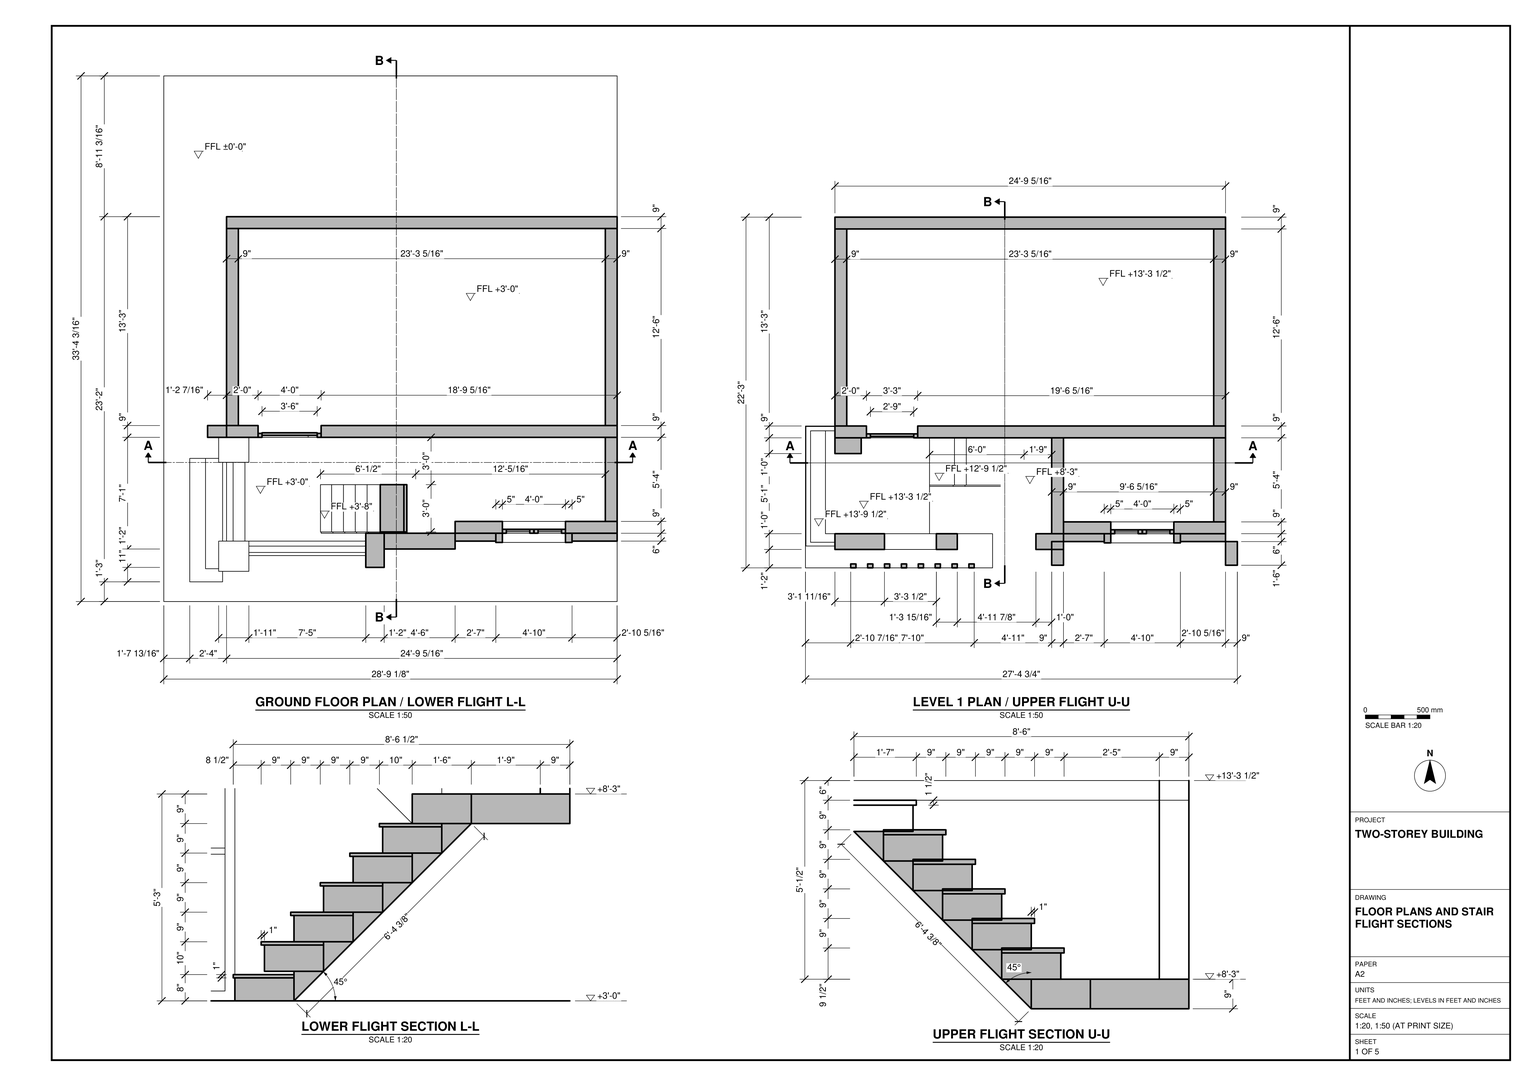
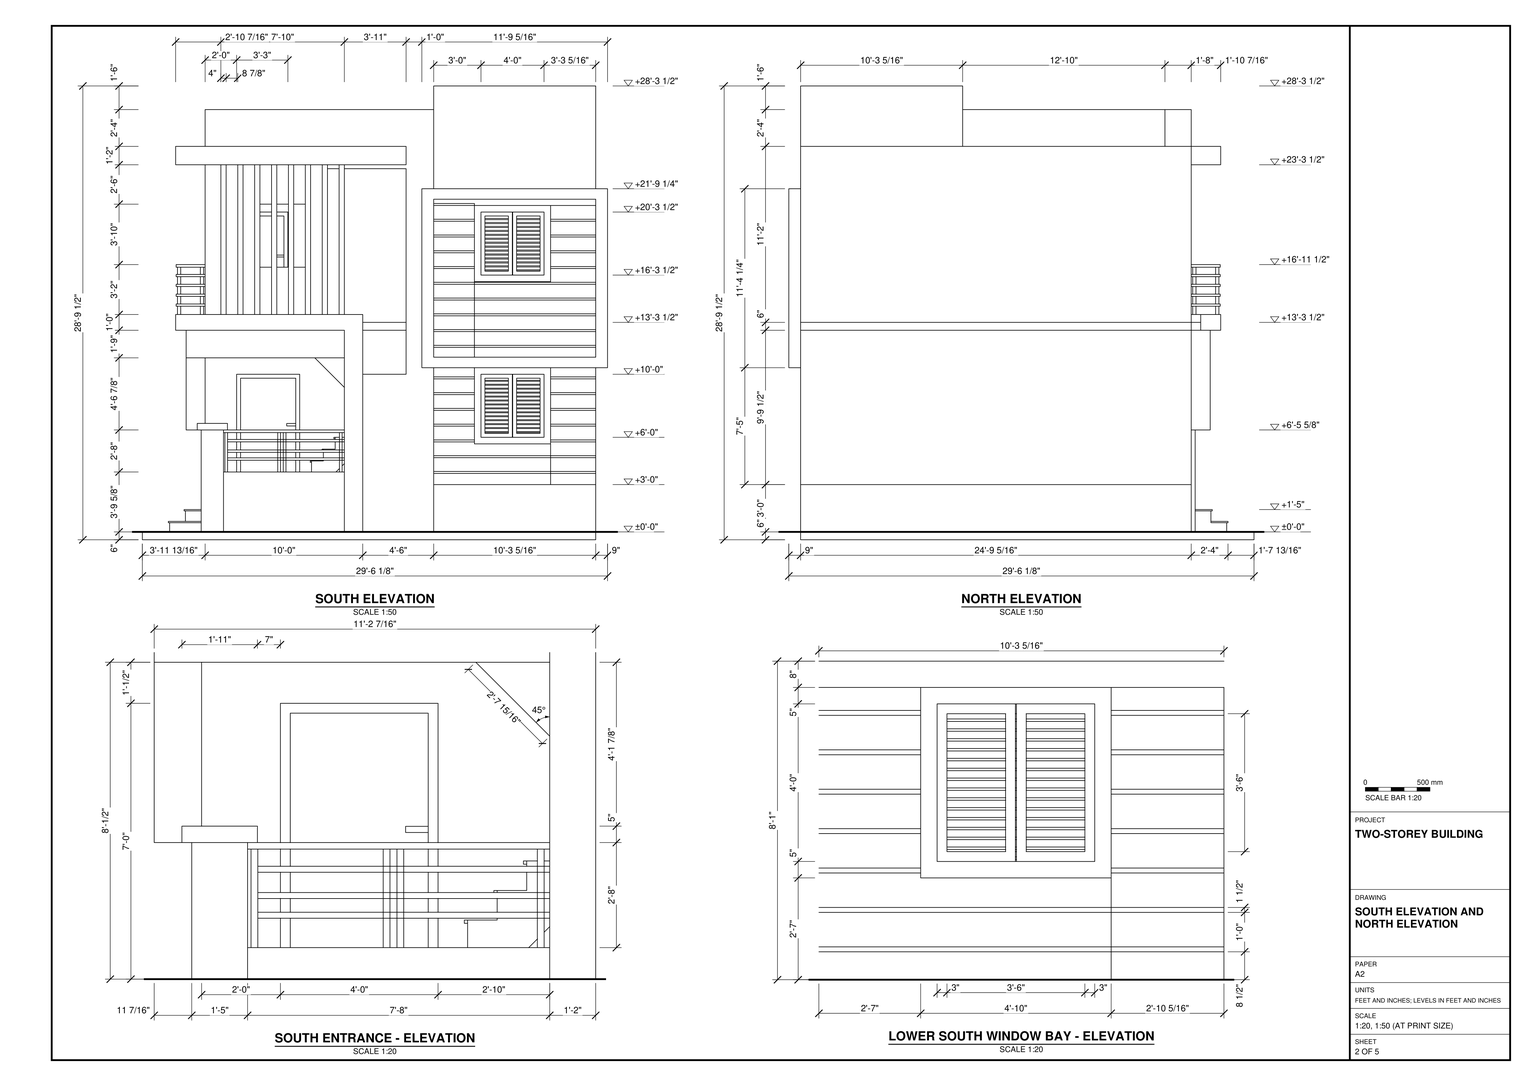
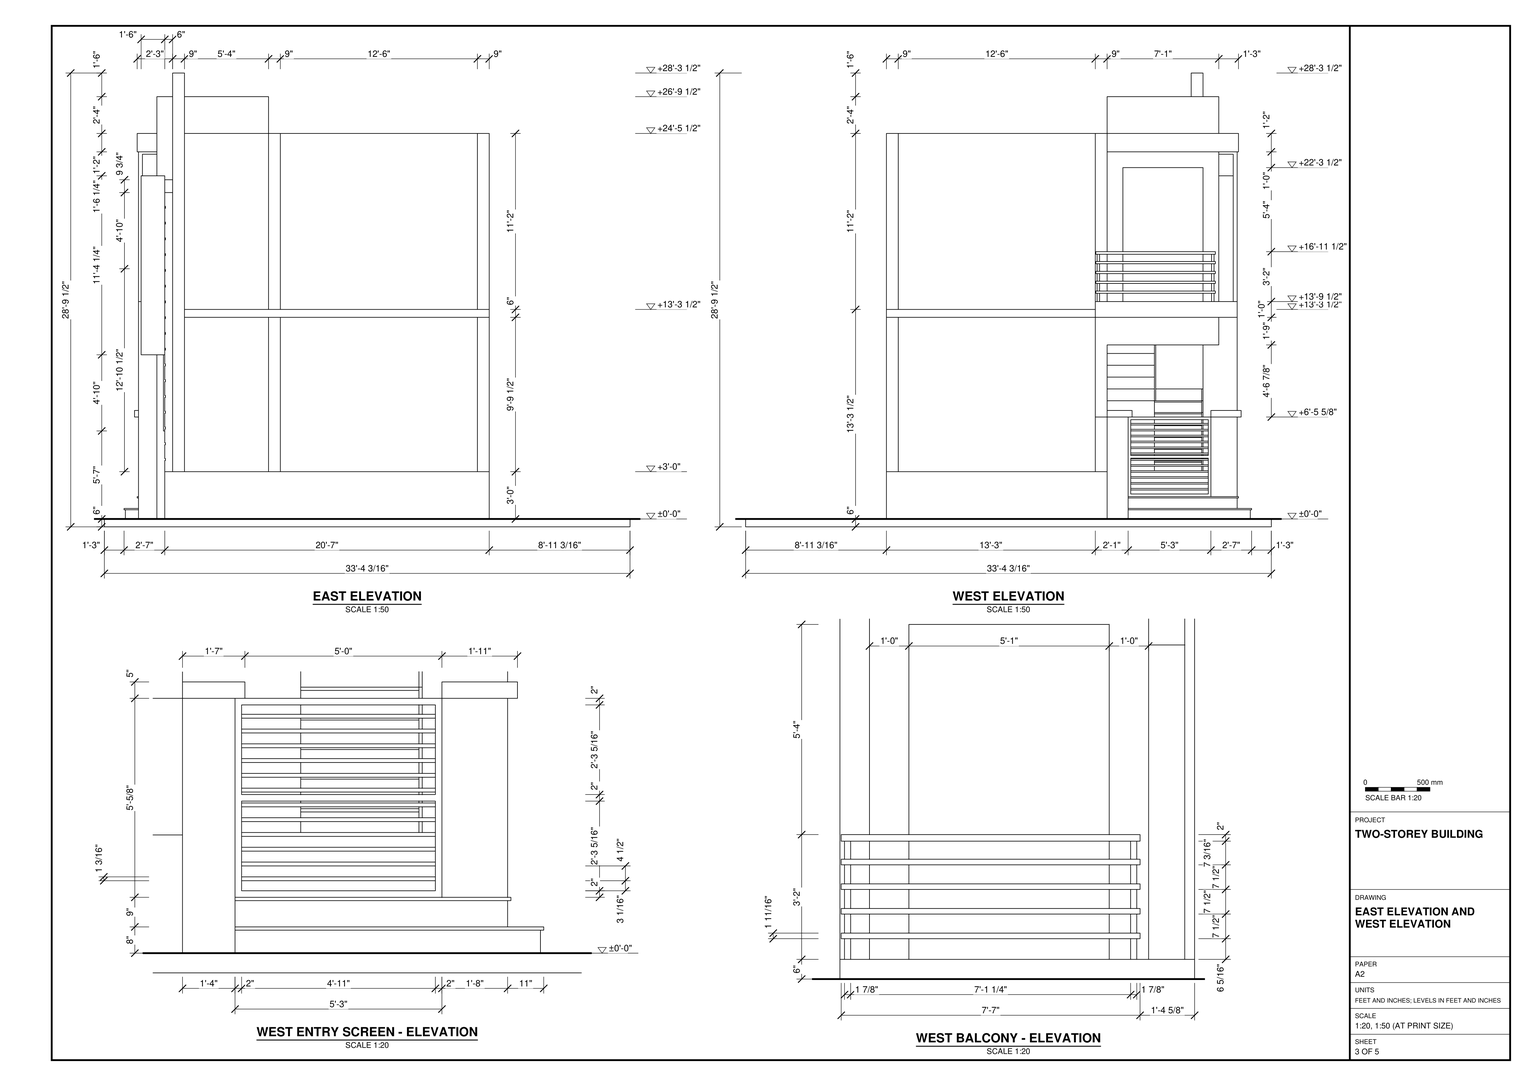
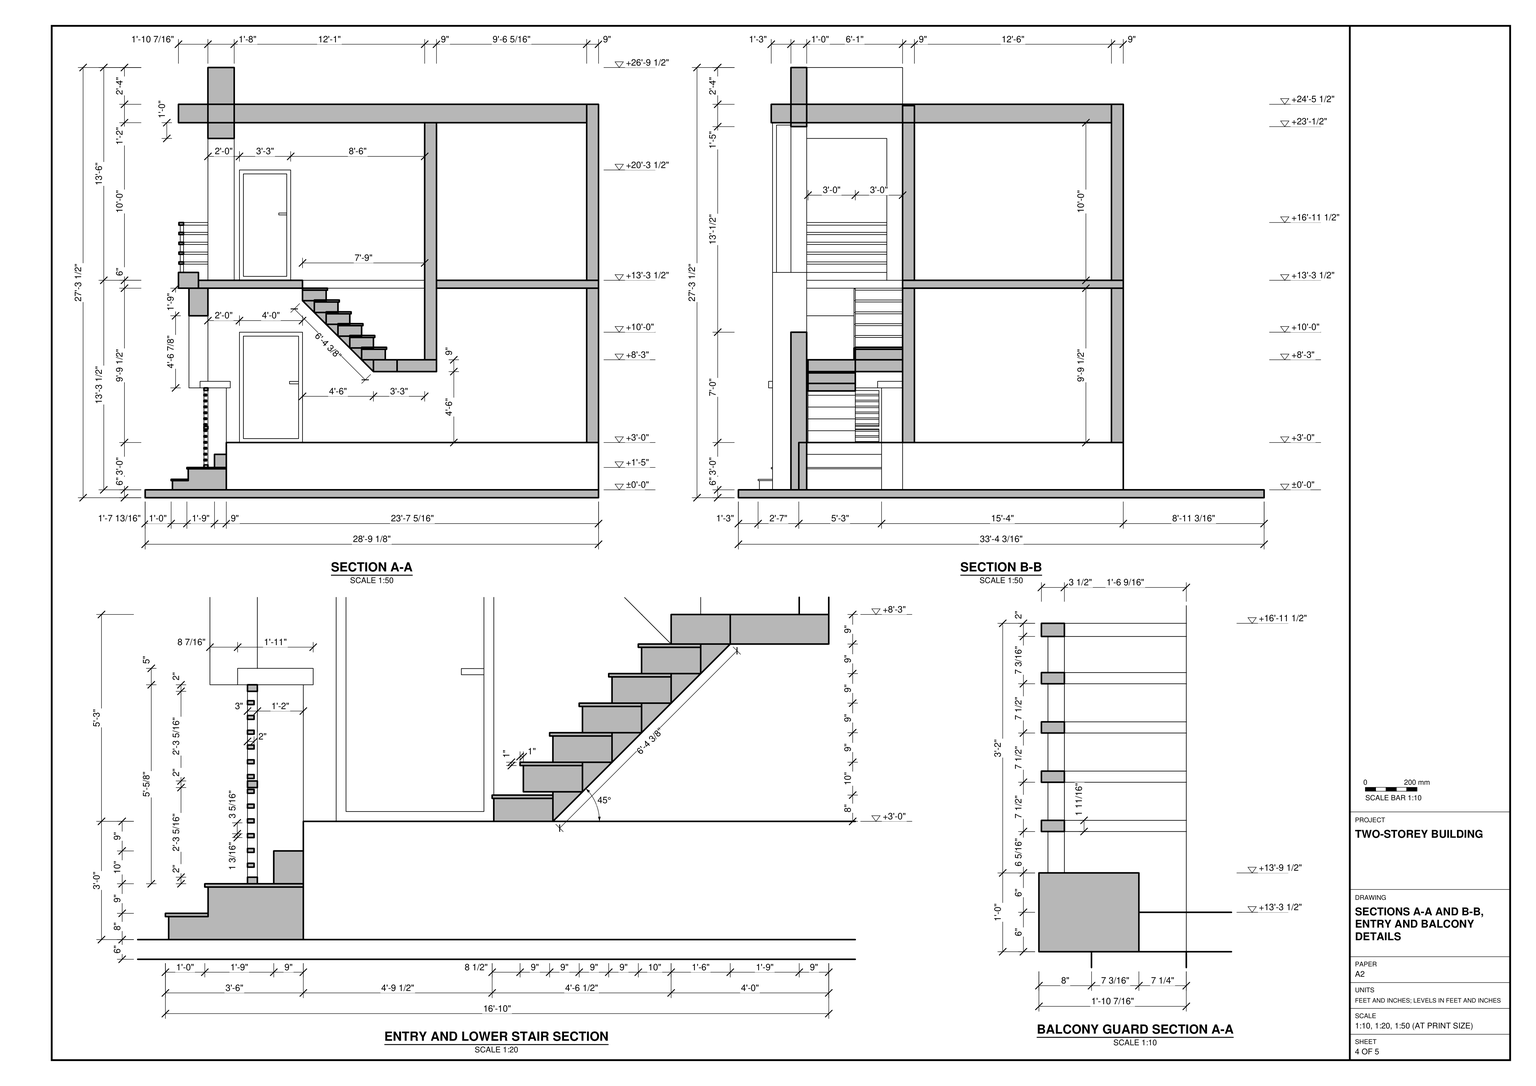
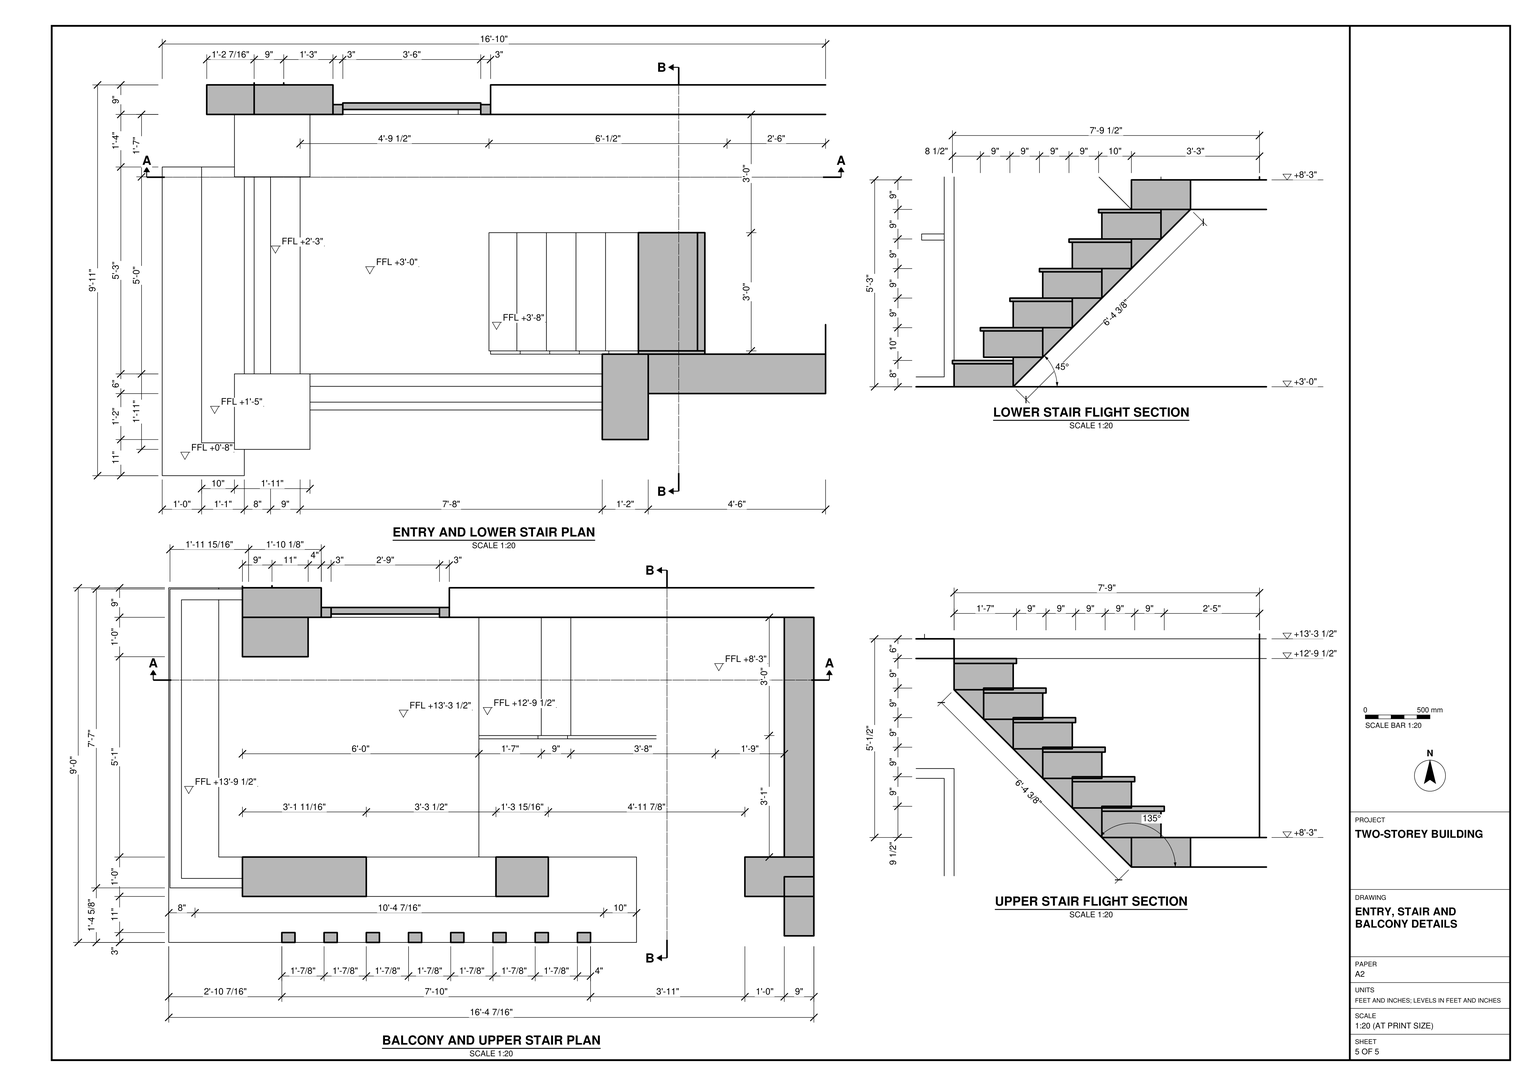
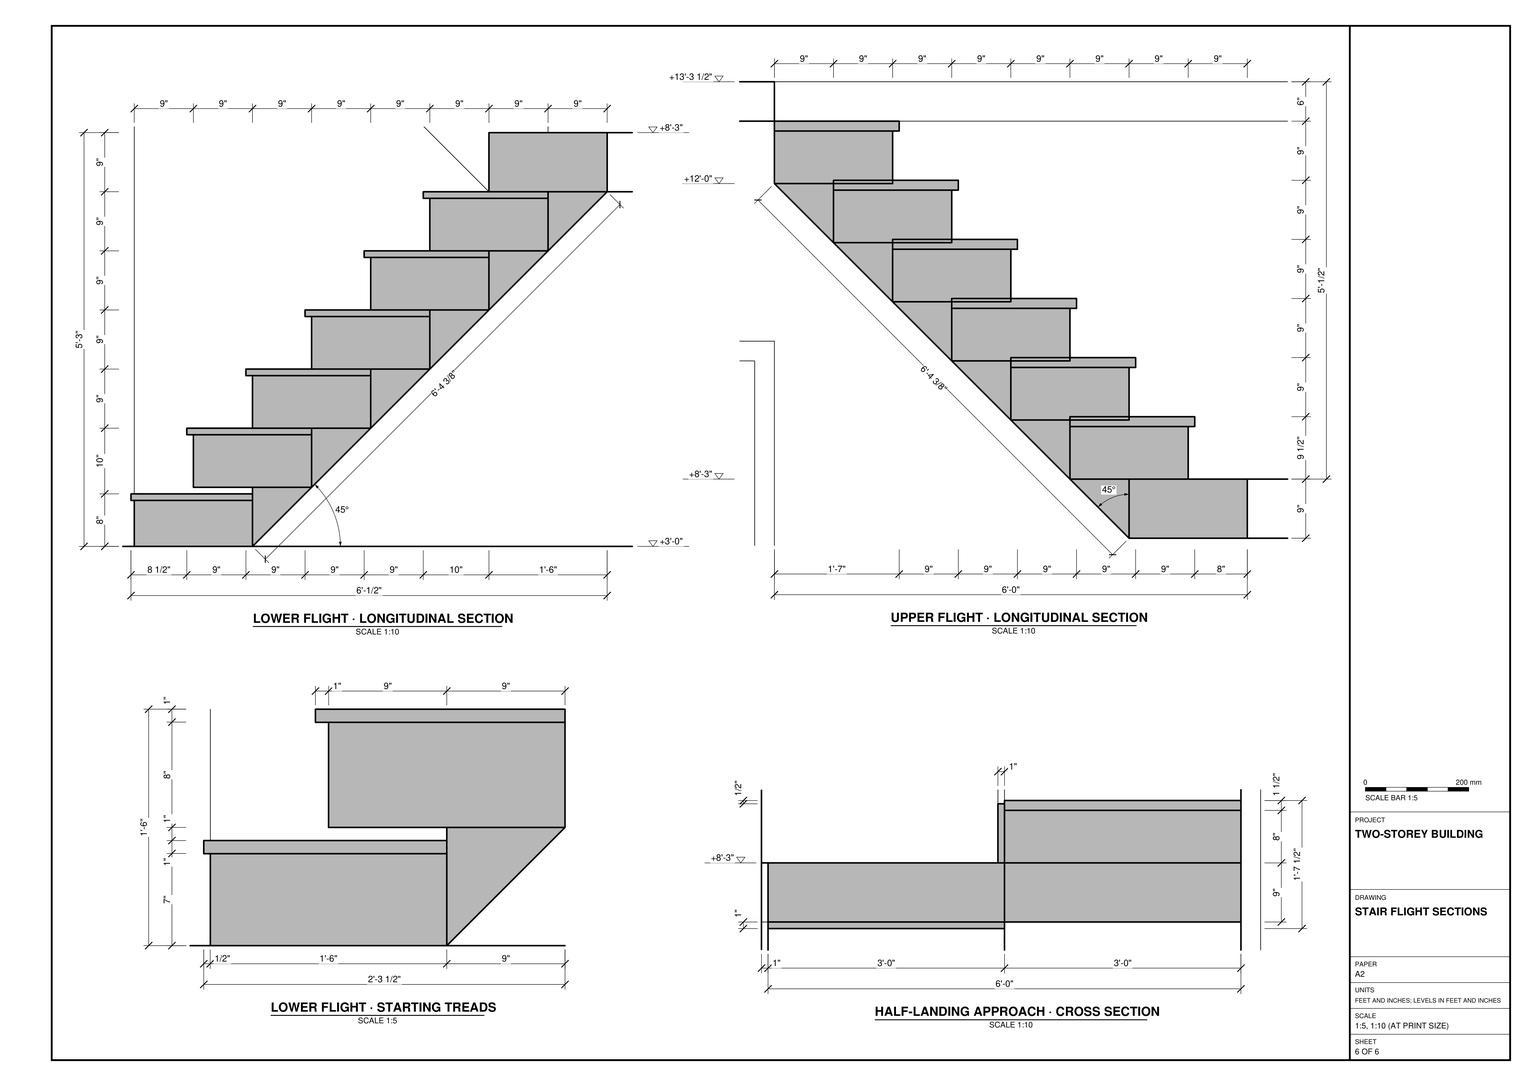
Build the two-storey building in SketchUp from task_files/diagram_01.pdf. Work in feet and inches. Set the overall width to 29'-6 1/8", depth to 33'-4 3/16" and height to 28'-9 1/2", including the base slab and projecting facade elements. Use ±0'-0" as the ground datum and +13'-3 1/2" as the upper storey level. Distinguish the ground datum from the raised lower floor at +3'-0".

Lay out the rectangular rear enclosure and the entrance, stair and window bay along its south side. Follow the wall thicknesses in plan, including the 9" walls around the rear enclosure. Model the base, raised floor, upper slab, balcony supports and flat roof profile with its changes in height. Use the flight sections to build the stair treads and risers, with the lower flight rising to the landing at +8'-3" and the upper flight returning to the upper floor.

Use the entrance and balcony details to position the steps, posts, horizontal rails and screens around the door openings. On the south window bay, model the stacked window units, horizontal bands and projecting upper surround. Keep the north elevation plain as drawn. Decor and loose items, if included, may be any suitable library components.

Keep shell elements such as walls, slabs and roof, and each furniture or joinery piece, in separate groups or components. Use components for repeated parts. Save one SketchUp model as output_files/two_storey_building_with_a_return_stair_and_balcony.skp.

# SketchUp Ruby script. Lengths in inches.
U = 1.inch
M = Sketchup.active_model
def pt(a) = Geom::Point3d.new(a.map { |v| v * U })
def face(e, loops, mat)
  f = e.add_face(loops[0].map { |a| pt(a) })
  loops[1..].each { |l| e.add_face(l.map { |a| pt(a) }).erase! }
  f.material = f.back_material = mat if mat
  f
end
# faces: each face lists its corners as indices into pts; further lists are holes
def faces(e, pts, list, mat = nil) = list.each { |f| face(e, (f[0].is_a?(Array) ? f : [f]).map { |l| l.map { |i| pts[i] } }, mat) }
# xy, xz, yz: faces in a plane at the given z, y or x. An outline is a flat list of corners, or four numbers for a rectangle; further outlines are holes
def ring(l) = l.size == 4 ? [[l[0], l[1]], [l[2], l[1]], [l[2], l[3]], [l[0], l[3]]] : l.each_slice(2).to_a
def flat(e, list, mat, &to3) = list.each { |f| face(e, (f[0].is_a?(Array) ? f : [f]).map { |l| ring(l).map { |u, v| to3.(u, v) } }, mat) }
def xy(e, z, list, mat = nil) = flat(e, list, mat) { |x, y| [x, y, z] }
def xz(e, y, list, mat = nil) = flat(e, list, mat) { |x, z| [x, y, z] }
def yz(e, x, list, mat = nil) = flat(e, list, mat) { |y, z| [x, y, z] }
def lines(e, pts, list) = list.each { |a, b| e.add_line(pt(pts[a]), pt(pts[b])) }
# prism: a flat outline (further loops are holes) pulled along v
def prism(e, loops, v, mat = nil)
  f = face(e, loops, mat); d = Geom::Vector3d.new(v.map { |x| x * U })
  f.pushpull(f.normal.samedirection?(d) ? d.length : -d.length)
end
def box(e, o, s, mat = nil) = prism(e, [[o, [o[0] + s[0], o[1], o[2]], [o[0] + s[0], o[1] + s[1], o[2]], [o[0], o[1] + s[1], o[2]]]], [0, 0, s[2]], mat)
def at(x, y, z, deg = 0) = Geom::Transformation.translation(pt([x, y, z])) * Geom::Transformation.rotation(ORIGIN, Z_AXIS, deg.degrees)
def axes(o, x, y, z) = Geom::Transformation.new([*x, 0, *y, 0, *z, 0, *pt(o).to_a, 1])
def part(name) = M.definitions.add(name)
# library, detail: a bought-in or finely detailed component or shape, given as its bounding box
def library(name, o, s) = part(name).tap { |d| box(d.entities, o, s) }
def detail(e, o, s) = box(e.add_group.entities, o, s)
def put(e, d, t, mat = nil) = e.add_instance(d, t).tap { |i| i.material = mat if mat }
def group(e, t, mat = nil) = e.add_group.tap { |g| g.transformation = t; g.material = mat if mat }.entities
root = M.entities
M.materials.add("[Color C08]").color = [109, 78, 39]
M.materials.add("[Color M04]").color = [142, 142, 142]
M.materials.add("[Wood Veneer 01]").color = [120, 70, 37]
c1 = part("Group\#36")
prism(c1.entities,[[[0,0.375,0],[0,0.28,0.01],[0,0.1875,0.05],[0,0.11,0.11],[0,0.05,0.1875],[0,0.01,0.28],[0,0,0.375],[0,0.01,0.47],[0,0.05,0.5625],[0,0.11,0.64],[0,0.1875,0.7],[0,0.28,0.74],[0,0.375,0.75],[0,0.47,0.74],[0,0.5625,0.7],[0,0.64,0.64],[0,0.7,0.5625],[0,0.74,0.47],[0,0.75,0.375],[0,0.74,0.28],[0,0.7,0.1875],[0,0.64,0.11],[0,0.5625,0.05],[0,0.47,0.01]]],[45,0,0])
c2 = part("Group\#47")
prism(c2.entities,[[[0,0.66,0.06],[0,0.55,0.01],[0,0.4375,0],[0,0.32,0.01],[0,0.22,0.06],[0,0.13,0.13],[0,0.06,0.22],[0,0.01,0.32],[0,0,0.4375],[0,0.01,0.55],[0,0.06,0.66],[0,0.13,0.75],[0,0.22,0.82],[0,0.32,0.86],[0,0.4375,0.875],[0,0.55,0.86],[0,0.66,0.82],[0,0.75,0.75],[0,0.82,0.66],[0,0.86,0.55],[0,0.875,0.4375],[0,0.86,0.32],[0,0.82,0.22],[0,0.75,0.13]]],[45,0,0])
c3 = part("Group\#62")
box(c3.entities,[0,0,0],[88.89,2,1.82])
c4 = part("Group\#72")
box(c4.entities,[0,0,-0.5],[2,59,1.18])
c5 = part("Group\#73")
box(c5.entities,[0,0,0],[2.5,1.875,36])
c6 = part("Group\#57")
prism(c6.entities,[[[0,3,0],[0,0,0],[0,0,114],[0,14,114],[0,14,112.1875],[0,3,112.1875]]],[4,0,0])
p = [[157.78,46,6],[157.78,46,42],[157.78,52,42],[59.78,40,291.5],[47.78,40,291.5],[47.78,125,291.5]]
lines(root,p,[[0,1],[1,2],[3,4],[4,5]])
g1 = group(root,at(-43.0625,-233.125,0))
box(g1,[43.0625,233.125,0],[345.125,400.1875,6])
g2 = group(root,at(47.78,53,6))
prism(g2,[[[297.34,240,0],[297.34,-7,0],[14,-7,0],[14,72,0],[0,72,0],[0,240,0]]],[0,0,36])
g3 = group(root,at(47.78,125,42))
prism(g3,[[[24,9,0],[0,9,0],[0,9,117.5],[297.34,9,117.5],[297.34,9,0],[72,9,0],[72,9,84],[24,9,84]]],[0,-9,0])
g4 = group(root,at(71.78,125,42),"[Wood Veneer 01]")
prism(g4,[[[0,3,0],[0,3,84],[48,3,84],[48,3,0]],[[3,3,81],[3,3,3],[45,3,3],[45,3,81]]],[0,-3,0])
g5 = group(root,at(74.78,126.5,45),"[Wood Veneer 01]")
box(g5,[0,0,0],[42,2,78])
g6 = group(root,at(110.91,124.5,86.66))
box(g6,[-1,0.5,0],[6.875,1.5,1.875])
g7 = group(root,at(119.78,53,42),"[Color M04]")
xy(g7,9,[[18,0,27,36]])
xy(g7,18,[[27,0,36,36]])
xy(g7,27,[[36,0,45,36]])
xy(g7,36,[[45,0,54,36]])
xy(g7,45,[[54,0,63,36]])
xy(g7,54,[[63,0,72,36]])
xz(g7,0,[[18,0,27,9,18,9],[27,9,36,18,27,18],[36,18,45,27,36,27],[45,27,54,36,45,36],[54,36,63,45,54,45],
  [63,45,72,54,63,54]])
xz(g7,36,[[18,0,18,9,27,9],[27,9,27,18,36,18],[36,18,36,27,45,27],[45,27,45,36,54,36],[54,36,54,45,63,45],
  [63,45,63,54,72,54]])
yz(g7,18,[[0,0,36,9]])
yz(g7,27,[[0,9,36,18]])
yz(g7,36,[[0,18,36,27]])
yz(g7,45,[[0,27,36,36]])
yz(g7,54,[[0,36,36,45]])
yz(g7,63,[[0,45,36,54]])
p = [[18,36,0],[27,36,9],[27,0,9],[18,0,0],[36,36,18],[36,0,18],
  [45,36,27],[45,0,27],[54,36,36],[54,0,36],[63,36,45],[63,0,45],
  [72,36,54],[72,0,54]]
faces(g7,p,[[0,1,2,3],[1,4,5,2],[4,6,7,5],[6,8,9,7],[8,10,11,9],[10,12,13,11]])
g8 = group(g7,at(9,0,9))
xy(g8,0,[[0,0,18,36]])
xy(g8,8,[[-1,0,0,36],[0,0,18,36]])
xy(g8,9,[[-1,0,18,36]])
xz(g8,0,[[0,0,18,8],[-1,8,18,9]])
xz(g8,36,[[0,0,18,8],[-1,8,18,9]])
yz(g8,-1,[[0,8,36,9]])
yz(g8,0,[[0,0,36,8]])
yz(g8,18,[[0,0,36,8],[0,8,36,9]])
g9 = group(g7,at(27,0,27))
xy(g9,0,[[0,0,18,36]])
xy(g9,8,[[-1,0,0,36],[0,0,18,36]])
xy(g9,9,[[-1,0,18,36]])
xz(g9,0,[[0,0,18,8],[-1,8,18,9]])
xz(g9,36,[[0,0,18,8],[-1,8,18,9]])
yz(g9,-1,[[0,8,36,9]])
yz(g9,0,[[0,0,36,8]])
yz(g9,18,[[0,0,36,8],[0,8,36,9]])
g10 = group(g7,at(18,0,18))
xy(g10,0,[[0,0,18,36]])
xy(g10,8,[[-1,0,0,36],[0,0,18,36]])
xy(g10,9,[[-1,0,18,36]])
xz(g10,0,[[0,0,18,8],[-1,8,18,9]])
xz(g10,36,[[0,0,18,8],[-1,8,18,9]])
yz(g10,-1,[[0,8,36,9]])
yz(g10,0,[[0,0,36,8]])
yz(g10,18,[[0,0,36,8],[0,8,36,9]])
g11 = group(g7,at(36,0,36))
xy(g11,0,[[0,0,18,36]])
xy(g11,8,[[-1,0,0,36],[0,0,18,36]])
xy(g11,9,[[-1,0,18,36]])
xz(g11,0,[[0,0,18,8],[-1,8,18,9]])
xz(g11,36,[[0,0,18,8],[-1,8,18,9]])
yz(g11,-1,[[0,8,36,9]])
yz(g11,0,[[0,0,36,8]])
yz(g11,18,[[0,0,36,8],[0,8,36,9]])
g12 = group(g7,at(54,0,54))
box(g12,[0,0,0],[18,36,9])
g13 = group(g7,at(0,0,0))
xy(g13,0,[[0,0,18,36]])
xy(g13,7,[[-0.5,0,0,36],[0,0,18,36]])
xy(g13,8,[[-0.5,0,18,36]])
xz(g13,0,[[0,0,18,7],[-0.5,7,18,8]])
xz(g13,36,[[0,0,18,7],[-0.5,7,18,8]])
yz(g13,-0.5,[[0,7,36,8]])
yz(g13,0,[[0,0,36,7]])
yz(g13,18,[[0,0,36,7],[0,7,36,8]])
g14 = group(g7,at(45,0,45))
xy(g14,0,[[0,0,18,36]])
xy(g14,8,[[-1,0,0,36],[0,0,18,36]])
xy(g14,9,[[-1,0,18,36]])
xz(g14,0,[[0,0,18,8],[-1,8,18,9]])
xz(g14,36,[[0,0,18,8],[-1,8,18,9]])
yz(g14,-1,[[0,8,36,9]])
yz(g14,0,[[0,0,36,8]])
yz(g14,18,[[0,0,36,8],[0,8,36,9]])
g15 = group(root,at(191.78,125,96,-180))
xy(g15,9,[[18,0,27,36]])
xy(g15,18,[[27,0,36,36]])
xy(g15,27,[[36,0,45,36]])
xy(g15,36,[[45,0,54,36]])
xy(g15,45,[[54,0,63,36]])
xy(g15,54,[[63,0,72,36]])
xz(g15,0,[[18,0,27,9,18,9],[27,9,36,18,27,18],[36,18,45,27,36,27],[45,27,54,36,45,36],[54,36,63,45,54,45],
  [63,45,72,54,63,54]])
xz(g15,36,[[18,0,18,9,27,9],[27,9,27,18,36,18],[36,18,36,27,45,27],[45,27,45,36,54,36],[54,36,54,45,63,45],
  [63,45,63,54,72,54]])
yz(g15,18,[[0,0,36,9]])
yz(g15,27,[[0,9,36,18]])
yz(g15,36,[[0,18,36,27]])
yz(g15,45,[[0,27,36,36]])
yz(g15,54,[[0,36,36,45]])
yz(g15,63,[[0,45,36,54]])
p = [[18,36,0],[27,36,9],[27,0,9],[18,0,0],[36,36,18],[36,0,18],
  [45,36,27],[45,0,27],[54,36,36],[54,0,36],[63,36,45],[63,0,45],
  [72,36,54],[72,0,54]]
faces(g15,p,[[0,1,2,3],[1,4,5,2],[4,6,7,5],[6,8,9,7],[8,10,11,9],[10,12,13,11]])
g16 = group(g15,at(9,0,9))
xy(g16,0,[[0,0,18,36]])
xy(g16,8,[[-1,0,0,36],[0,0,18,36]])
xy(g16,9.5,[[-1,0,18,36]])
xz(g16,0,[[0,0,18,8],[-1,8,18,9.5]])
xz(g16,36,[[0,0,18,8],[-1,8,18,9.5]])
yz(g16,-1,[[0,8,36,9.5]])
yz(g16,0,[[0,0,36,8]])
yz(g16,18,[[0,0,36,8],[0,8,36,9.5]])
g17 = group(g15,at(27,0,27))
xy(g17,0,[[0,0,18,36]])
xy(g17,8,[[-1,0,0,36],[0,0,18,36]])
xy(g17,9.5,[[-1,0,18,36]])
xz(g17,0,[[0,0,18,8],[-1,8,18,9.5]])
xz(g17,36,[[0,0,18,8],[-1,8,18,9.5]])
yz(g17,-1,[[0,8,36,9.5]])
yz(g17,0,[[0,0,36,8]])
yz(g17,18,[[0,0,36,8],[0,8,36,9.5]])
g18 = group(g15,at(18,0,18))
xy(g18,0,[[0,0,18,36]])
xy(g18,8,[[-1,0,0,36],[0,0,18,36]])
xy(g18,9.5,[[-1,0,18,36]])
xz(g18,0,[[0,0,18,8],[-1,8,18,9.5]])
xz(g18,36,[[0,0,18,8],[-1,8,18,9.5]])
yz(g18,-1,[[0,8,36,9.5]])
yz(g18,0,[[0,0,36,8]])
yz(g18,18,[[0,0,36,8],[0,8,36,9.5]])
g19 = group(g15,at(36,0,36))
xy(g19,0,[[0,0,18,36]])
xy(g19,8,[[-1,0,0,36],[0,0,18,36]])
xy(g19,9.5,[[-1,0,18,36]])
xz(g19,0,[[0,0,18,8],[-1,8,18,9.5]])
xz(g19,36,[[0,0,18,8],[-1,8,18,9.5]])
yz(g19,-1,[[0,8,36,9.5]])
yz(g19,0,[[0,0,36,8]])
yz(g19,18,[[0,0,36,8],[0,8,36,9.5]])
g20 = group(g15,at(0,0,0))
box(g20,[0,0,0],[18,36,9])
g21 = group(g15,at(45,0,45))
xy(g21,0,[[0,0,18,36]])
xy(g21,8,[[-1,0,0,36],[0,0,18,36]])
xy(g21,9.5,[[-1,0,18,36]])
xz(g21,0,[[0,0,18,8],[-1,8,18,9.5]])
xz(g21,36,[[0,0,18,8],[-1,8,18,9.5]])
yz(g21,-1,[[0,8,36,9.5]])
yz(g21,0,[[0,0,36,8]])
yz(g21,18,[[0,0,36,8],[0,8,36,9.5]])
g22 = group(root,at(191.78,53,96))
box(g22,[0,0,0],[30,72,9])
g23 = group(root,at(119.78,88,96))
prism(g23,[[[0,1,63],[18,1,63],[18,1,54],[27,1,54],[27,1,45],[36,1,45],[36,1,36],[45,1,36],[45,1,27],[54,1,27],[54,1,18],[63,1,18],[63,1,9],[54,1,9],[54,1,0],[0,1,54]]],[0,-1,0])
g24 = group(root,at(119.78,52,42))
prism(g24,[[[0,1,9],[9,1,9],[9,1,18],[18,1,18],[18,1,27],[27,1,27],[27,1,36],[36,1,36],[36,1,45],[45,1,45],[45,1,54],[54,1,54],[54,1,63],[102,1,63],[102,1,54],[72,1,54],[18,1,0],[0,1,0]]],[0,-1,0])
g25 = group(root,at(119.78,89,150))
xy(g25,0,[[0,0,18,36]])
xy(g25,8,[[0,0,18,36],[18,0,19,36]])
xy(g25,9.5,[[0,0,19,36]])
xz(g25,0,[[0,0,18,8],[0,8,19,9.5]])
xz(g25,36,[[0,0,18,8],[0,8,19,9.5]])
yz(g25,0,[[0,0,36,8],[0,8,36,9.5]])
yz(g25,18,[[0,0,36,8]])
yz(g25,19,[[0,8,36,9.5]])
g26 = group(root,at(47.78,284,42))
box(g26,[0,0,0],[297.34,9,117.5])
g27 = group(root,at(47.78,134,42))
box(g27,[0,0,0],[9,150,117.5])
g28 = group(root,at(336.125,134,42))
box(g28,[0,0,0],[9,150,117.5])
g29 = group(root,at(47.78,125,159.5))
g30 = group(g29,at(0,-85,0))
prism(g30,[[[297.34,253,0],[297.34,21,0],[174,21,0],[174,85,0],[72,85,0],[72,12,0],[-7.22,12,0],[-7.22,94,0],[0,94,0],[0,253,0]]],[0,0,6])
g31 = group(g29,at(288.34,-64,-117.5))
box(g31,[0,0,0],[9,64,117.5])
g32 = group(root,at(221.78,52,42))
prism(g32,[[[123.34,9,0],[0,9,0],[0,9,303.5],[123.34,9,303.5]],[[36,9,36],[84,9,36],[84,9,84],[36,9,84]],[[84,9,207.5],[36,9,207.5],[36,9,159.5],[84,9,159.5]]],[0,-9,0])
g33 = group(root,at(252.78,47,73))
prism(g33,[[[0,-2,58],[0,-2,0],[58,-2,0],[58,-2,58]],[[5,-2,5],[5,-2,53],[53,-2,53],[53,-2,5]]],[0,7,0])
g34 = group(root,at(257.78,52,78),"[Wood Veneer 01]")
prism(g34,[[[24.15,0,0],[48,0,0],[48,0,48],[24.15,0,48]],[[27.15,0,3],[27.15,0,45],[45,0,45],[45,0,3]]],[0,3,0])
prism(g34,[[[23.85,0,48],[0,0,48],[0,0,0],[23.85,0,0]],[[20.85,0,3],[3,0,3],[3,0,45],[20.85,0,45]]],[0,3,0])
p = [[24.15,3,0],[23.85,3,0],[23.85,3,48],[24.15,3,48]]
lines(g34,p,[[0,1],[2,3]])
put(root,c1,at(260.78,53.125,120.65),"[Wood Veneer 01]")
put(root,c1,at(260.78,53.125,117.65),"[Wood Veneer 01]")
put(root,c1,at(260.78,53.125,114.65),"[Wood Veneer 01]")
put(root,c1,at(260.78,53.125,111.65),"[Wood Veneer 01]")
put(root,c1,at(260.78,53.125,108.65),"[Wood Veneer 01]")
put(root,c1,at(260.78,53.125,105.65),"[Wood Veneer 01]")
put(root,c1,at(260.78,53.125,102.65),"[Wood Veneer 01]")
put(root,c1,at(260.78,53.125,99.65),"[Wood Veneer 01]")
put(root,c1,at(260.78,53.125,96.65),"[Wood Veneer 01]")
put(root,c1,at(260.78,53.125,93.65),"[Wood Veneer 01]")
put(root,c1,at(260.78,53.125,90.65),"[Wood Veneer 01]")
put(root,c1,at(260.78,53.125,87.65),"[Wood Veneer 01]")
put(root,c1,at(260.78,53.125,84.65),"[Wood Veneer 01]")
put(root,c1,at(260.78,53.125,81.65),"[Wood Veneer 01]")
put(root,c1,at(260.78,53.125,78.65))
put(root,c1,at(260.78,53.125,75.65))
g35 = group(root,at(260.78,55,81),"[Wood Veneer 01]")
xz(g35,0,[[0,0,42,42]])
g36 = group(root,at(47.78,125,165.5))
prism(g36,[[[297.34,9,0],[63,9,0],[63,9,84],[24,9,84],[24,9,0],[0,9,0],[0,9,134],[9,9,134],[9,9,133],[288.34,9,133],[288.34,9,134],[297.34,9,134]]],[0,-9,0])
g37 = group(root,at(71.78,125,165.5),"[Wood Veneer 01]")
prism(g37,[[[0,3,0],[0,3,84],[39,3,84],[39,3,0]],[[3,3,3],[36,3,3],[36,3,81],[3,3,81]]],[0,-3,0])
g38 = group(root,at(74.78,126,168.5),"[Wood Veneer 01]")
box(g38,[0,0,0],[33,2,78])
g39 = group(root,at(101.72,125,215.28))
box(g39,[0,0,0],[6.0625,1,1.4375])
g40 = group(root,at(47.78,284,165.5))
box(g40,[0,0,0],[297.34,9,134])
g41 = group(root,at(336.125,134,165.5))
box(g41,[0,0,0],[9,150,134])
g42 = group(root,at(47.78,134,165.5))
box(g42,[0,0,0],[9,150,134])
g43 = group(root,at(252.78,47,196.5))
prism(g43,[[[0,5,58],[58,5,58],[58,5,0],[0,5,0]],[[5,5,5],[53,5,5],[53,5,53],[5,5,53]]],[0,-7,0])
g44 = group(root,at(257.78,52,201.5),"[Wood Veneer 01]")
prism(g44,[[[23.85,3,48],[23.85,3,0],[0,3,0],[0,3,48]],[[20.85,3,3],[20.85,3,45],[3,3,45],[3,3,3]]],[0,-3,0])
prism(g44,[[[48,3,0],[24.15,3,0],[24.15,3,48],[48,3,48]],[[45,3,45],[27.15,3,45],[27.15,3,3],[45,3,3]]],[0,-3,0])
p = [[24.15,3,0],[23.85,3,0],[23.85,3,48],[24.15,3,48]]
lines(g44,p,[[0,1],[2,3]])
put(root,c2,at(260.78,53.0625,243.7),"[Wood Veneer 01]")
put(root,c2,at(260.78,53.0625,240.7),"[Wood Veneer 01]")
put(root,c2,at(260.78,53.0625,237.7),"[Wood Veneer 01]")
put(root,c2,at(260.78,53.0625,234.7),"[Wood Veneer 01]")
put(root,c2,at(260.78,53.0625,231.7),"[Wood Veneer 01]")
put(root,c2,at(260.78,53.0625,228.7),"[Wood Veneer 01]")
put(root,c2,at(260.78,53.0625,225.7),"[Wood Veneer 01]")
put(root,c2,at(260.78,53.0625,222.7),"[Wood Veneer 01]")
put(root,c2,at(260.78,53.0625,219.7),"[Wood Veneer 01]")
put(root,c2,at(260.78,53.0625,216.7),"[Wood Veneer 01]")
put(root,c2,at(260.78,53.0625,213.7),"[Wood Veneer 01]")
put(root,c2,at(260.78,53.0625,210.7),"[Wood Veneer 01]")
put(root,c2,at(260.78,53.0625,207.7),"[Wood Veneer 01]")
put(root,c2,at(260.78,53.0625,204.7),"[Wood Veneer 01]")
g45 = group(root,at(260.78,55,204.5),"[Wood Veneer 01]")
xz(g45,0,[[0,0,42,42]])
g46 = group(root,at(336.125,61,165.5))
box(g46,[0,0,0],[9,64,134])
g47 = group(root,at(221.78,46,42),"[Color M04]")
xy(g47,0,[[0,0,31,6],[31,0,89,6]])
xy(g47,8.5,[[0,0,89,0.5]])
xy(g47,10,[[0,0,89,0.5]])
xy(g47,20.5,[[0,0,89,0.5]])
xy(g47,22,[[0,0,89,0.5]])
xy(g47,31,[[31,0,89,6]])
xy(g47,32.5,[[0,0,31,0.5]])
xy(g47,34,[[0,0,31,0.5]])
xy(g47,44.5,[[0,0,31,0.5]])
xy(g47,46,[[0,0,31,0.5]])
xy(g47,56.5,[[0,0,31,0.5]])
xy(g47,58,[[0,0,31,0.5]])
xy(g47,68.5,[[0,0,31,0.5]])
xy(g47,70,[[0,0,31,0.5]])
xy(g47,80.5,[[0,0,31,0.5]])
xy(g47,82,[[0,0,31,0.5]])
xy(g47,92.5,[[0,0,31,0.5]])
xy(g47,94,[[0,0,31,0.5]])
xy(g47,104.5,[[0,0,31,0.5]])
xy(g47,106,[[0,0,31,0.5]])
xy(g47,116.5,[[0,0,31,0.5]])
xy(g47,118,[[0,0,31,0.5]])
xy(g47,128.5,[[0,0,31,0.5]])
xy(g47,130,[[0,0,31,0.5]])
xy(g47,140.5,[[0,0,31,0.5]])
xy(g47,142,[[0,0,31,0.5]])
xy(g47,152.5,[[0,0,31,0.5]])
xy(g47,154,[[0,0,31,0.5]])
xy(g47,164.5,[[0,0,31,0.5]])
xy(g47,166,[[0,0,31,0.5]])
xy(g47,176.5,[[0,0,31,0.5]])
xy(g47,178,[[0,0,31,0.5]])
xy(g47,188.5,[[0,0,31,0.5]])
xy(g47,190,[[0,0,31,0.5]])
xy(g47,200.5,[[0,0,31,0.5]])
xy(g47,202,[[0,0,31,0.5]])
xy(g47,212.5,[[0,0,31,0.5],[31,0,123.34,6]])
xy(g47,214,[[0,0,31,0.5]])
xy(g47,222.25,[[0,0,123.34,6]])
xz(g47,0,[[0,0,89,8.5],[0,10,89,20.5],[0,22,89,22,89,31,31,31,31,32.5,0,32.5],[0,34,31,44.5],[0,46,31,56.5],
  [0,58,31,68.5],[0,70,31,80.5],[0,82,31,92.5],[0,94,31,104.5],[0,106,31,116.5],
  [0,118,31,128.5],[0,130,31,140.5],[0,142,31,152.5],[0,154,31,164.5],[0,166,31,176.5],
  [0,178,31,188.5],[0,190,31,200.5],[0,202,31,212.5],[31,212.5,123.34,212.5,123.34,222.25,0,222.25,0,214,31,214]])
xz(g47,0.5,[[0,8.5,89,10],[0,20.5,89,22],[0,32.5,31,34],[0,44.5,31,46],[0,56.5,31,58],
  [0,68.5,31,70],[0,80.5,31,82],[0,92.5,31,94],[0,104.5,31,106],[0,116.5,31,118],
  [0,128.5,31,130],[0,140.5,31,142],[0,152.5,31,154],[0,164.5,31,166],[0,176.5,31,178],
  [0,188.5,31,190],[0,200.5,31,202],[0,212.5,31,214]])
xz(g47,6,[[0,0,0,222.25,123.34,222.25,123.34,212.5,31,212.5,31,0],[31,0,89,31]])
yz(g47,0,[[0,0,0,8.5,0.5,8.5,0.5,10,0,10,0,20.5,0.5,20.5,0.5,22,0,22,0,32.5,0.5,32.5,0.5,34,0,34,0,44.5,0.5,44.5,0.5,46,0,46,0,56.5,0.5,56.5,0.5,58,0,58,0,68.5,0.5,68.5,0.5,70,0,70,0,80.5,0.5,80.5,0.5,82,0,82,0,92.5,0.5,92.5,0.5,94,0,94,0,104.5,0.5,104.5,0.5,106,0,106,0,116.5,0.5,116.5,0.5,118,0,118,0,128.5,0.5,128.5,0.5,130,0,130,0,140.5,0.5,140.5,0.5,142,0,142,0,152.5,0.5,152.5,0.5,154,0,154,0,164.5,0.5,164.5,0.5,166,0,166,0,176.5,0.5,176.5,0.5,178,0,178,0,188.5,0.5,188.5,0.5,190,0,190,0,200.5,0.5,200.5,0.5,202,0,202,0,212.5,0.5,212.5,0.5,214,0,214,0,222.25,6,222.25,6,0]])
yz(g47,31,[[0,31,6,31,6,212.5,0,212.5,0,202,0.5,202,0.5,200.5,0,200.5,0,190,0.5,190,0.5,188.5,0,188.5,0,178,0.5,178,0.5,176.5,0,176.5,0,166,0.5,166,0.5,164.5,0,164.5,0,154,0.5,154,0.5,152.5,0,152.5,0,142,0.5,142,0.5,140.5,0,140.5,0,130,0.5,130,0.5,128.5,0,128.5,0,118,0.5,118,0.5,116.5,0,116.5,0,106,0.5,106,0.5,104.5,0,104.5,0,94,0.5,94,0.5,92.5,0,92.5,0,82,0.5,82,0.5,80.5,0,80.5,0,70,0.5,70,0.5,68.5,0,68.5,0,58,0.5,58,0.5,56.5,0,56.5,0,46,0.5,46,0.5,44.5,0,44.5,0,34,0.5,34,0.5,32.5,0,32.5],[0,212.5,0.5,214]])
yz(g47,89,[[0,0,6,0,6,31,0,31,0,22,0.5,22,0.5,20.5,0,20.5,0,10,0.5,10,0.5,8.5,0,8.5]])
yz(g47,123.34,[[0,212.5,6,222.25]])
g48 = group(root,at(249.78,46,42))
xy(g48,0,[[61,0,95.34,6]])
xy(g48,8.5,[[61,0,95.34,0.5]])
xy(g48,10,[[61,0,95.34,0.5]])
xy(g48,20.5,[[61,0,95.34,0.5]])
xy(g48,22,[[61,0,95.34,0.5]])
xy(g48,32.5,[[61,0,95.34,0.5]])
xy(g48,34,[[61,0,95.34,0.5]])
xy(g48,44.5,[[61,0,95.34,0.5]])
xy(g48,46,[[61,0,95.34,0.5]])
xy(g48,56.5,[[61,0,95.34,0.5]])
xy(g48,58,[[61,0,95.34,0.5]])
xy(g48,68.5,[[61,0,95.34,0.5]])
xy(g48,70,[[61,0,95.34,0.5]])
xy(g48,80.5,[[61,0,95.34,0.5]])
xy(g48,82,[[61,0,95.34,0.5]])
xy(g48,89,[[3,0,61,6]])
xy(g48,92.5,[[3,0,95.34,0.5]])
xy(g48,94,[[3,0,95.34,0.5]])
xy(g48,104.5,[[3,0,95.34,0.5]])
xy(g48,106,[[3,0,95.34,0.5]])
xy(g48,116.5,[[3,0,95.34,0.5]])
xy(g48,118,[[3,0,95.34,0.5]])
xy(g48,128.5,[[3,0,95.34,0.5]])
xy(g48,130,[[3,0,95.34,0.5]])
xy(g48,140.5,[[3,0,95.34,0.5]])
xy(g48,142,[[3,0,95.34,0.5]])
xy(g48,152.5,[[3,0,95.34,0.5]])
xy(g48,154,[[3,0,95.34,0.5]])
xy(g48,154.5,[[3,0,61,6]])
xy(g48,164.5,[[61,0,95.34,0.5]])
xy(g48,166,[[61,0,95.34,0.5]])
xy(g48,176.5,[[61,0,95.34,0.5]])
xy(g48,178,[[61,0,95.34,0.5]])
xy(g48,188.5,[[61,0,95.34,0.5]])
xy(g48,190,[[61,0,95.34,0.5]])
xy(g48,200.5,[[61,0,95.34,0.5]])
xy(g48,202,[[61,0,95.34,0.5]])
xy(g48,212.5,[[61,0,95.34,0.5],[61,0.5,95.34,6]])
xz(g48,0,[[61,0,95.34,8.5],[61,10,95.34,20.5],[61,22,95.34,32.5],[61,34,95.34,44.5],[61,46,95.34,56.5],
  [61,58,95.34,68.5],[61,70,95.34,80.5],[61,82,95.34,82,95.34,92.5,3,92.5,3,89,61,89],[3,94,95.34,104.5],[3,106,95.34,116.5],
  [3,118,95.34,128.5],[3,130,95.34,140.5],[3,142,95.34,152.5],[3,154,95.34,154,95.34,164.5,61,164.5,61,154.5,3,154.5],[61,166,95.34,176.5],
  [61,178,95.34,188.5],[61,190,95.34,200.5],[61,202,95.34,212.5]])
xz(g48,0.5,[[61,8.5,95.34,10],[61,20.5,95.34,22],[61,32.5,95.34,34],[61,44.5,95.34,46],[61,56.5,95.34,58],
  [61,68.5,95.34,70],[61,80.5,95.34,82],[3,92.5,95.34,94],[3,104.5,95.34,106],[3,116.5,95.34,118],
  [3,128.5,95.34,130],[3,140.5,95.34,142],[3,152.5,95.34,154],[61,164.5,95.34,166],[61,176.5,95.34,178],
  [61,188.5,95.34,190],[61,200.5,95.34,202]])
xz(g48,6,[[61,0,61,89,3,89,3,154.5,61,154.5,61,212.5,95.34,212.5,95.34,0]])
yz(g48,3,[[0,89,0,92.5,0.5,92.5,0.5,94,0,94,0,104.5,0.5,104.5,0.5,106,0,106,0,116.5,0.5,116.5,0.5,118,0,118,0,128.5,0.5,128.5,0.5,130,0,130,0,140.5,0.5,140.5,0.5,142,0,142,0,152.5,0.5,152.5,0.5,154,0,154,0,154.5,6,154.5,6,89]])
yz(g48,61,[[0,0,0,8.5,0.5,8.5,0.5,10,0,10,0,20.5,0.5,20.5,0.5,22,0,22,0,32.5,0.5,32.5,0.5,34,0,34,0,44.5,0.5,44.5,0.5,46,0,46,0,56.5,0.5,56.5,0.5,58,0,58,0,68.5,0.5,68.5,0.5,70,0,70,0,80.5,0.5,80.5,0.5,82,0,82,0,89,6,89,6,0],[0,154.5,0,164.5,0.5,164.5,0.5,166,0,166,0,176.5,0.5,176.5,0.5,178,0,178,0,188.5,0.5,188.5,0.5,190,0,190,0,200.5,0.5,200.5,0.5,202,0,202,0,212.5,6,212.5,6,154.5]])
yz(g48,95.34,[[0,0,6,0,6,212.5,0,212.5,0,202,0.5,202,0.5,200.5,0,200.5,0,190,0.5,190,0.5,188.5,0,188.5,0,178,0.5,178,0.5,176.5,0,176.5,0,166,0.5,166,0.5,164.5,0,164.5,0,154,0.5,154,0.5,152.5,0,152.5,0,142,0.5,142,0.5,140.5,0,140.5,0,130,0.5,130,0.5,128.5,0,128.5,0,118,0.5,118,0.5,116.5,0,116.5,0,106,0.5,106,0.5,104.5,0,104.5,0,94,0.5,94,0.5,92.5,0,92.5,0,82,0.5,82,0.5,80.5,0,80.5,0,70,0.5,70,0.5,68.5,0,68.5,0,58,0.5,58,0.5,56.5,0,56.5,0,46,0.5,46,0.5,44.5,0,44.5,0,34,0.5,34,0.5,32.5,0,32.5,0,22,0.5,22,0.5,20.5,0,20.5,0,10,0.5,10,0.5,8.5,0,8.5]])
g49 = group(root,at(212.78,28,131))
prism(g49,[[[141.34,18,136.25],[141.34,18,0],[0,18,0],[0,18,136.25]],[[9,18,128.25],[9,18,8],[132.34,18,8],[132.34,18,128.25]]],[0,-18,0])
g50 = group(root,at(212.78,52,105))
box(g50,[0,0,0],[9,73,180.5])
g51 = group(root,at(47.78,125,285.5))
prism(g51,[[[288.34,159,0],[288.34,-64,0],[174,-64,0],[174,-73,0],[153,-73,0],[153,-100,0],[-22.4375,-100,0],[-22.4375,0,0],[9,0,0],[9,159,0]]],[0,0,14])
g52 = group(root,at(23.78,38,6))
xy(g52,0,[[130,-12,144,14]])
xy(g52,153.5,[[1.5625,-12,1.5625,96,16.78,96,16.78,14,130,14,130,-12]])
xy(g52,165.5,[[1.5625,-12,144,-12,144,14,16.78,14,16.78,96,1.5625,96]])
xz(g52,-12,[[130,0,144,0,144,165.5,1.5625,165.5,1.5625,153.5,130,153.5]])
xz(g52,14,[[130,0,130,153.5,16.78,153.5,16.78,165.5,144,165.5,144,0]])
xz(g52,96,[[1.5625,153.5,16.78,165.5]])
yz(g52,1.5625,[[-12,153.5,96,165.5]])
yz(g52,16.78,[[14,153.5,96,165.5]])
yz(g52,130,[[-12,0,14,153.5]])
yz(g52,144,[[-12,0,14,165.5]])
g53 = group(root,at(33.35,52,87.3))
xy(g53,-3.7,[[0,73,14.4375,82]])
xy(g53,51.2,[[0,-12,0,73,14.4375,73,14.4375,-5.02,124.4375,-5.02,124.4375,-12]])
xy(g53,72.2,[[0,-12,124.4375,-12,124.4375,-5.02,14.4375,-5.02,14.4375,82,0,82]])
xz(g53,-12,[[0,51.2,124.4375,72.2]])
xz(g53,-5.02,[[14.4375,51.2,124.4375,72.2]])
xz(g53,73,[[0,-3.7,14.4375,51.2]])
xz(g53,82,[[0,-3.7,14.4375,72.2]])
yz(g53,0,[[73,-3.7,73,51.2,-12,51.2,-12,72.2,82,72.2,82,-3.7]])
yz(g53,14.4375,[[73,-3.7,82,-3.7,82,72.2,-5.02,72.2,-5.02,51.2,73,51.2]])
yz(g53,124.4375,[[-12,51.2,-5.02,72.2]])
g54 = group(root,at(47.78,40,6),"[Color C08]")
xy(g54,0,[[120,0,174,12]])
xy(g54,120,[[120,0,153,12]])
xy(g54,153.5,[[0,73,20,85]])
xy(g54,165.5,[[0,0,93.14,12]])
xy(g54,201.5,[[37.71,0,77.2,12]])
xy(g54,249.5,[[37.71,0,77.2,12]])
xy(g54,267.5,[[0,12,20,73]])
xy(g54,276.5,[[93.14,0,153,12]])
xy(g54,321.5,[[0,0,174,0,174,12,20,12,20,85,0,85]])
xz(g54,0,[[[120,0,174,0,174,125,165,125,165,258.25,174,258.25,174,321.5,0,321.5,0,165.5,93.14,165.5,93.14,276.5,153,276.5,153,120,120,120],[37.71,201.5,77.2,249.5]],[165,125,174,258.25]])
xz(g54,12,[[120,0,120,120,153,120,153,285.5,20,285.5,20,321.5,174,321.5,174,0],[[0,165.5,93.14,267.5],[37.71,201.5,77.2,249.5]],[20,267.5,93.14,276.5],[20,276.5,153,285.5]])
xz(g54,73,[[0,153.5,20,267.5]])
xz(g54,85,[[0,153.5,20,321.5]])
yz(g54,0,[[73,153.5,73,267.5,12,267.5,12,165.5,0,165.5,0,321.5,85,321.5,85,153.5]])
yz(g54,20,[[73,153.5,85,153.5,85,321.5,12,321.5,12,267.5,73,267.5]])
yz(g54,37.71,[[0,201.5,12,249.5]])
yz(g54,77.2,[[0,201.5,12,249.5]])
yz(g54,93.14,[[0,165.5,12,276.5]])
yz(g54,120,[[0,0,12,120]])
yz(g54,153,[[0,120,12,276.5]])
yz(g54,174,[[0,0,12,321.5]])
p = [[174,0,258.25],[174,6,258.25],[174,0,125],[174,6,125]]
lines(g54,p,[[0,1],[2,3]])
g55 = group(root,at(44.78,26,6))
box(g55,[0,0,0],[17,20,77.6])
g56 = group(root,at(61.78,35,6))
box(g56,[0,0,0],[92,11,45.6])
g57 = group(root,at(62.83,38.38,51.6))
box(g57,[0,0,0],[2.0625,3.8125,30])
g58 = group(root,at(103.08,38.38,51.6))
box(g58,[0,0.1,0],[2.0625,3.71,30])
g59 = group(root,at(107.27,38.38,51.6))
box(g59,[0,0.1,0],[2.0625,3.71,30])
g60 = group(root,at(150.02,38.38,51.6))
box(g60,[0,0.1,0],[2.0625,3.71,30])
g61 = group(root,at(61.78,37.38,81.6))
box(g61,[0,0,0],[92,4.8125,2])
put(root,c3,at(64.89,38.38,74.55))
put(root,c3,at(64.89,38.38,66.55))
put(root,c3,at(64.89,38.38,60.55))
g62 = group(root,at(41.78,23,83.6))
box(g62,[0,0,0],[23,23,5])
g63 = group(root,at(44.78,105,6),"[Color M04]")
box(g63,[0,4,0],[17,16,77.6])
g64 = group(root,at(41.78,102,83.6))
box(g64,[0,4,0],[23,19,5])
g65 = group(root,at(20.78,16,6),"[Color M04]")
xy(g65,0,[[0,0,0,93,41,93,41,30,24,30,24,0]])
xy(g65,7,[[-1,-1,24,0],[-1,0,0,93],[0,0,24,0,24,10,12,10,12,93,0,93]])
xy(g65,8,[[-1,-1,24,-1,24,10,12,10,12,93,-1,93]])
xy(g65,16,[[11,9,24,10],[11,10,12,93],[12,10,24,10,24,30,41,30,41,93,12,93]])
xy(g65,17,[[11,9,24,9,24,30,41,30,41,93,11,93]])
xz(g65,-1,[[-1,7,24,8]])
xz(g65,0,[[0,0,24,7]])
xz(g65,9,[[11,16,24,17]])
xz(g65,10,[[12,7,24,8],[12,8,24,16]])
xz(g65,30,[[24,0,41,16],[24,16,41,17]])
xz(g65,93,[[0,0,0,7,12,7,12,16,41,16,41,0],[-1,7,12,8],[11,16,41,17]])
yz(g65,-1,[[-1,7,93,8]])
yz(g65,0,[[0,0,93,7]])
yz(g65,11,[[9,16,93,17]])
yz(g65,12,[[10,7,93,8],[10,8,93,16]])
yz(g65,24,[[0,0,30,0,30,16,10,16,10,7,0,7],[-1,7,10,8],[9,16,30,17]])
yz(g65,41,[[30,0,93,16],[30,16,93,17]])
p = [[24,10,24],[24,10,17]]
lines(g65,p,[[0,1]])
g66 = group(root,at(44.78,46,23))
box(g66,[8,0,0],[9,63,10])
g67 = group(root,at(44.78,46,23))
prism(g67,[[[0,0,60.6],[0,63,60.6],[0,63,0],[0,0,0]],[[0,2,31.3],[0,61,31.3],[0,61,58.6],[0,2,58.6]],[[0,61,2],[0,61,29.3],[0,2,29.3],[0,2,2]]],[3,0,0])
put(root,c4,at(44.78,48,78.0625))
put(root,c4,at(44.78,48,73.5625))
put(root,c4,at(44.78,48,69.0625))
put(root,c4,at(44.78,48,64.5625))
put(root,c4,at(44.78,48,60.0625))
put(root,c4,at(44.78,48,55.5625))
put(root,c4,at(44.78,48,51.0625))
put(root,c4,at(44.78,48,46.5625))
put(root,c4,at(44.78,48,42.0625))
put(root,c4,at(44.78,48,37.5625))
put(root,c4,at(44.78,48,33.0625))
put(root,c4,at(44.78,48,28.5625))
put(root,c5,at(44.16,43.61,171.5))
put(root,c5,at(26.72,43.61,171.5))
put(root,c5,at(26.72,130.73,171.5))
g68 = group(root,at(59.78,26,171.5))
put(g68,c6,at(64.29,0,0))
put(g68,c6,at(38.57,0,0))
put(g68,c6,at(25.71,0,0))
put(g68,c6,at(12.86,0,0))
put(g68,c6,at(51.43,0,0))
put(g68,c6,at(90,0,0))
put(g68,c6,at(77.14,0,0))
put(g68,c6,at(0,0,0))
g69 = group(root,at(25.72,42.61,177.8))
g70 = group(g69,at(0,0,7.2))
prism(g70,[[[0,91,0.3],[23.9375,91,0.3],[23.9375,87.72,0.3],[3.5,87.72,0.3],[3.5,2.875,0.3],[23.9375,2.875,0.3],[23.9375,0,0.3],[0,0,0.3]]],[0,0,1.7])
g71 = group(g69,at(0,0,-0.3))
prism(g71,[[[0,91,0.3],[23.9375,91,0.3],[23.9375,87.72,0.3],[3.5,87.72,0.3],[3.5,2.875,0.3],[23.9375,2.875,0.3],[23.9375,0,0.3],[0,0,0.3]]],[0,0,1.7])
g72 = group(g69,at(0,0,14.7))
prism(g72,[[[0,91,0.3],[23.9375,91,0.3],[23.9375,87.72,0.3],[3.5,87.72,0.3],[3.5,2.875,0.3],[23.9375,2.875,0.3],[23.9375,0,0.3],[0,0,0.3]]],[0,0,1.7])
g73 = group(g69,at(0,0,29.7))
prism(g73,[[[0,91,0],[23.9375,91,0],[23.9375,87.72,0],[3.5,87.72,0],[3.5,2.875,0],[23.9375,2.875,0],[23.9375,0,0],[0,0,0]]],[0,0,2])
g74 = group(g69,at(0,0,22.2))
prism(g74,[[[0,91,0.3],[23.9375,91,0.3],[23.9375,87.72,0.3],[3.5,87.72,0.3],[3.5,2.875,0.3],[23.9375,2.875,0.3],[23.9375,0,0.3],[0,0,0.3]]],[0,0,1.7])
